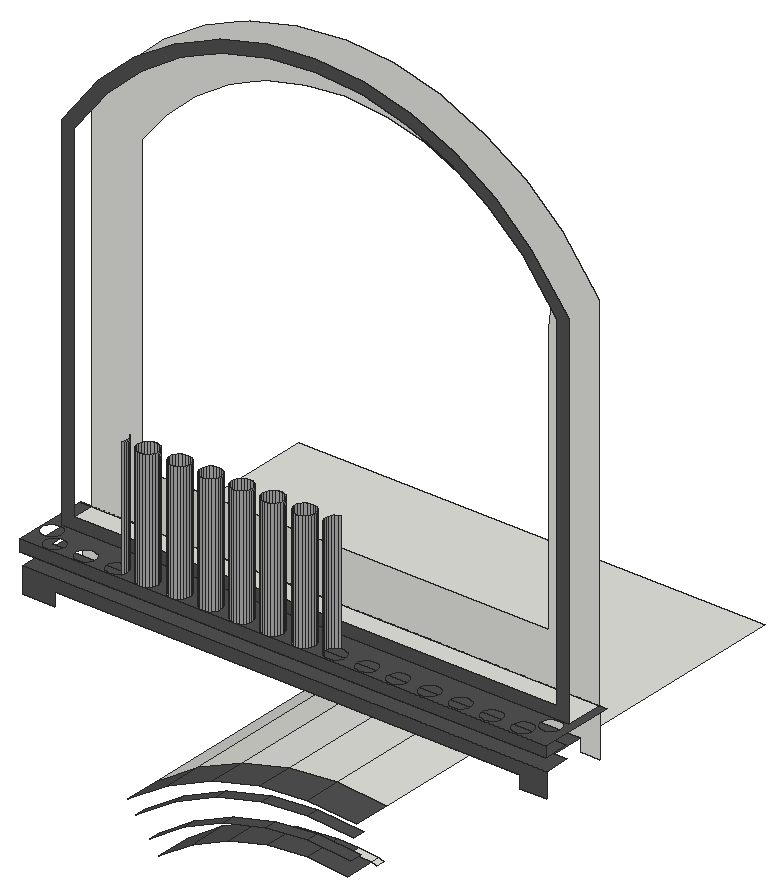
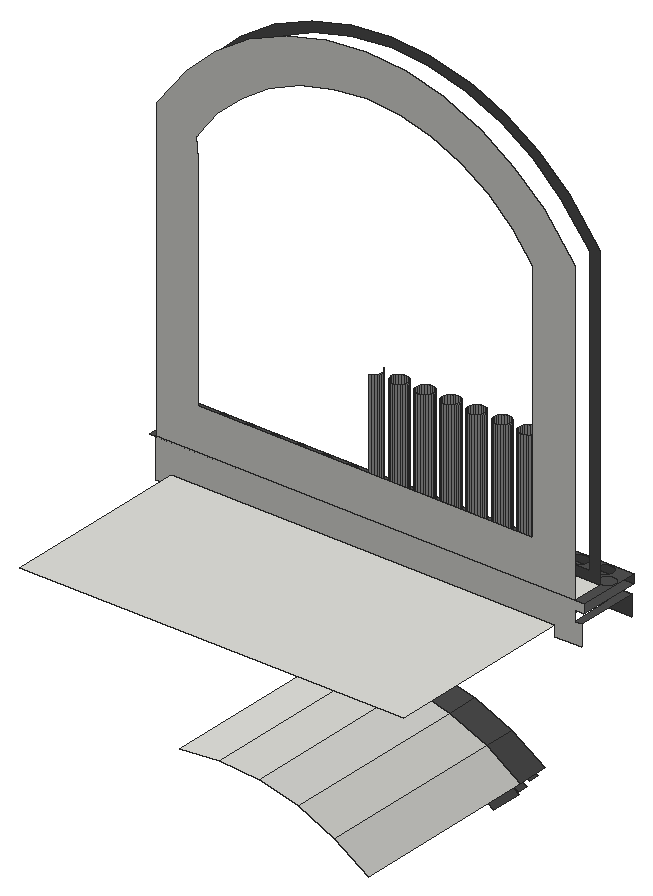
# SketchUp Ruby script. Lengths in inches.
U = 1.inch
M = Sketchup.active_model
def pt(a) = Geom::Point3d.new(a.map { |v| v * U })
def face(e, loops, mat)
  f = e.add_face(loops[0].map { |a| pt(a) })
  loops[1..].each { |l| e.add_face(l.map { |a| pt(a) }).erase! }
  f.material = f.back_material = mat if mat
  f
end
# faces: each face lists its corners as indices into pts; further lists are holes
def faces(e, pts, list, mat = nil) = list.each { |f| face(e, (f[0].is_a?(Array) ? f : [f]).map { |l| l.map { |i| pts[i] } }, mat) }
# xy, xz, yz: faces in a plane at the given z, y or x. An outline is a flat list of corners, or four numbers for a rectangle; further outlines are holes
def ring(l) = l.size == 4 ? [[l[0], l[1]], [l[2], l[1]], [l[2], l[3]], [l[0], l[3]]] : l.each_slice(2).to_a
def flat(e, list, mat, &to3) = list.each { |f| face(e, (f[0].is_a?(Array) ? f : [f]).map { |l| ring(l).map { |u, v| to3.(u, v) } }, mat) }
def xy(e, z, list, mat = nil) = flat(e, list, mat) { |x, y| [x, y, z] }
def xz(e, y, list, mat = nil) = flat(e, list, mat) { |x, z| [x, y, z] }
def yz(e, x, list, mat = nil) = flat(e, list, mat) { |y, z| [x, y, z] }
def lines(e, pts, list) = list.each { |a, b| e.add_line(pt(pts[a]), pt(pts[b])) }
# prism: a flat outline (further loops are holes) pulled along v
def prism(e, loops, v, mat = nil)
  f = face(e, loops, mat); d = Geom::Vector3d.new(v.map { |x| x * U })
  f.pushpull(f.normal.samedirection?(d) ? d.length : -d.length)
end
def box(e, o, s, mat = nil) = prism(e, [[o, [o[0] + s[0], o[1], o[2]], [o[0] + s[0], o[1] + s[1], o[2]], [o[0], o[1] + s[1], o[2]]]], [0, 0, s[2]], mat)
def at(x, y, z, deg = 0) = Geom::Transformation.translation(pt([x, y, z])) * Geom::Transformation.rotation(ORIGIN, Z_AXIS, deg.degrees)
def axes(o, x, y, z) = Geom::Transformation.new([*x, 0, *y, 0, *z, 0, *pt(o).to_a, 1])
def part(name) = M.definitions.add(name)
# library, detail: a bought-in or finely detailed component or shape, given as its bounding box
def library(name, o, s) = part(name).tap { |d| box(d.entities, o, s) }
def detail(e, o, s) = box(e.add_group.entities, o, s)
def put(e, d, t, mat = nil) = e.add_instance(d, t).tap { |i| i.material = mat if mat }
def group(e, t, mat = nil) = e.add_group.tap { |g| g.transformation = t; g.material = mat if mat }.entities
root = M.entities
M.materials.add("[0132_LightGray]").color = [169, 169, 169]
M.materials.add("[0135_DarkGray]").color = [81, 81, 81]
xy(root,487.28,[[247.74,49.6875,358.5,104.375]])
xy(root,487.28,[[247.74,31.6875,358.5,49.6875]],"[0135_DarkGray]")
xy(root,490.18,[[240.07,31.6875,364.76,31.6875,364.76,37.6875,242.14,37.6875,242.14,49.6875,240.07,49.6875]],"[0135_DarkGray]")
xy(root,493.07,[[239.45,31.6875,239.45,49.6875,242.14,49.6875,242.14,37.6875,364.64,37.6875,364.64,31.6875]],"[0135_DarkGray]")
xy(root,495.66,[[267.85,31.88,267.22,31.96,266.63,32.21,266.13,32.6,265.74,33.1,265.5,33.6875,265.41,34.32,265.5,34.95,265.74,35.54,266.13,36.04,266.63,36.43,267.22,36.67,267.85,36.76,268.48,36.67,269.07,36.43,269.58,36.04,269.96,35.54,270.21,34.95,270.29,34.32,270.21,33.6875,269.96,33.1,269.58,32.6,269.07,32.21,268.48,31.96],[275.29,31.88,274.66,31.96,274.07,32.21,273.57,32.6,273.18,33.1,272.93,33.6875,272.85,34.32,272.93,34.95,273.18,35.54,273.57,36.04,274.07,36.43,274.66,36.67,275.29,36.76,275.92,36.67,276.51,36.43,277.01,36.04,277.4,35.54,277.64,34.95,277.73,34.32,277.64,33.6875,277.4,33.1,277.01,32.6,276.51,32.21,275.92,31.96],[282.73,31.88,282.1,31.96,281.51,32.21,281,32.6,280.62,33.1,280.37,33.6875,280.29,34.32,280.37,34.95,280.62,35.54,281,36.04,281.51,36.43,282.1,36.67,282.73,36.76,283.36,36.67,283.95,36.43,284.45,36.04,284.84,35.54,285.08,34.95,285.16,34.32,285.08,33.6875,284.84,33.1,284.45,32.6,283.95,32.21,283.36,31.96],[290.16,31.88,289.53,31.96,288.95,32.21,288.44,32.6,288.05,33.1,287.81,33.6875,287.73,34.32,287.81,34.95,288.05,35.54,288.44,36.04,288.95,36.43,289.53,36.67,290.16,36.76,290.79,36.67,291.38,36.43,291.89,36.04,292.28,35.54,292.52,34.95,292.6,34.32,292.52,33.6875,292.28,33.1,291.89,32.6,291.38,32.21,290.79,31.96],[297.6,31.88,296.97,31.96,296.38,32.21,295.88,32.6,295.49,33.1,295.25,33.6875,295.16,34.32,295.25,34.95,295.49,35.54,295.88,36.04,296.38,36.43,296.97,36.67,297.6,36.76,298.23,36.67,298.82,36.43,299.33,36.04,299.71,35.54,299.96,34.95,300.04,34.32,299.96,33.6875,299.71,33.1,299.33,32.6,298.82,32.21,298.23,31.96],
  [305.04,31.88,304.41,31.96,303.82,32.21,303.32,32.6,302.93,33.1,302.68,33.6875,302.6,34.32,302.68,34.95,302.93,35.54,303.32,36.04,303.82,36.43,304.41,36.67,305.04,36.76,305.67,36.67,306.26,36.43,306.76,36.04,307.15,35.54,307.39,34.95,307.48,34.32,307.39,33.6875,307.15,33.1,306.76,32.6,306.26,32.21,305.67,31.96],[242.14,40.6875,362.82,49.6875]])
xy(root,495.66,[[[239.45,31.6875,364.64,31.6875,364.64,49.6875,362.82,49.6875,362.82,40.6875,242.14,40.6875,242.14,49.6875,239.45,49.6875],[245.54,31.88,244.91,31.96,244.32,32.21,243.82,32.6,243.43,33.1,243.18,33.6875,243.1,34.32,243.18,34.95,243.43,35.54,243.82,36.04,244.32,36.43,244.91,36.67,245.54,36.76,246.17,36.67,246.76,36.43,247.26,36.04,247.65,35.54,247.89,34.95,247.98,34.32,247.89,33.6875,247.65,33.1,247.26,32.6,246.76,32.21,246.17,31.96],[252.98,31.88,252.35,31.96,251.76,32.21,251.25,32.6,250.87,33.1,250.62,33.6875,250.54,34.32,250.62,34.95,250.87,35.54,251.25,36.04,251.76,36.43,252.35,36.67,252.98,36.76,253.61,36.67,254.2,36.43,254.7,36.04,255.09,35.54,255.33,34.95,255.41,34.32,255.33,33.6875,255.09,33.1,254.7,32.6,254.2,32.21,253.61,31.96],[260.41,31.88,259.78,31.96,259.2,32.21,258.69,32.6,258.3,33.1,258.06,33.6875,257.98,34.32,258.06,34.95,258.3,35.54,258.69,36.04,259.2,36.43,259.78,36.67,260.41,36.76,261.04,36.67,261.63,36.43,262.14,36.04,262.53,35.54,262.77,34.95,262.85,34.32,262.77,33.6875,262.53,33.1,262.14,32.6,261.63,32.21,261.04,31.96],[267.85,31.88,267.22,31.96,266.63,32.21,266.13,32.6,265.74,33.1,265.5,33.6875,265.41,34.32,265.5,34.95,265.74,35.54,266.13,36.04,266.63,36.43,267.22,36.67,267.85,36.76,268.48,36.67,269.07,36.43,269.58,36.04,269.96,35.54,270.21,34.95,270.29,34.32,270.21,33.6875,269.96,33.1,269.58,32.6,269.07,32.21,268.48,31.96],[275.29,31.88,274.66,31.96,274.07,32.21,273.57,32.6,273.18,33.1,272.93,33.6875,272.85,34.32,272.93,34.95,273.18,35.54,273.57,36.04,274.07,36.43,274.66,36.67,275.29,36.76,275.92,36.67,276.51,36.43,277.01,36.04,277.4,35.54,277.64,34.95,277.73,34.32,277.64,33.6875,277.4,33.1,277.01,32.6,276.51,32.21,275.92,31.96],[282.73,31.88,282.1,31.96,281.51,32.21,281,32.6,280.62,33.1,280.37,33.6875,280.29,34.32,280.37,34.95,280.62,35.54,281,36.04,281.51,36.43,282.1,36.67,282.73,36.76,283.36,36.67,283.95,36.43,284.45,36.04,284.84,35.54,285.08,34.95,285.16,34.32,285.08,33.6875,284.84,33.1,284.45,32.6,283.95,32.21,283.36,31.96],[290.16,31.88,289.53,31.96,288.95,32.21,288.44,32.6,288.05,33.1,287.81,33.6875,287.73,34.32,287.81,34.95,288.05,35.54,288.44,36.04,288.95,36.43,289.53,36.67,290.16,36.76,290.79,36.67,291.38,36.43,291.89,36.04,292.28,35.54,292.52,34.95,292.6,34.32,292.52,33.6875,292.28,33.1,291.89,32.6,291.38,32.21,290.79,31.96],[297.6,31.88,296.97,31.96,296.38,32.21,295.88,32.6,295.49,33.1,295.25,33.6875,295.16,34.32,295.25,34.95,295.49,35.54,295.88,36.04,296.38,36.43,296.97,36.67,297.6,36.76,298.23,36.67,298.82,36.43,299.33,36.04,299.71,35.54,299.96,34.95,300.04,34.32,299.96,33.6875,299.71,33.1,299.33,32.6,298.82,32.21,298.23,31.96],[305.04,31.88,304.41,31.96,303.82,32.21,303.32,32.6,302.93,33.1,302.68,33.6875,302.6,34.32,302.68,34.95,302.93,35.54,303.32,36.04,303.82,36.43,304.41,36.67,305.04,36.76,305.67,36.67,306.26,36.43,306.76,36.04,307.15,35.54,307.39,34.95,307.48,34.32,307.39,33.6875,307.15,33.1,306.76,32.6,306.26,32.21,305.67,31.96],[312.48,31.88,311.85,31.96,311.26,32.21,310.75,32.6,310.37,33.1,310.12,33.6875,310.04,34.32,310.12,34.95,310.37,35.54,310.75,36.04,311.26,36.43,311.85,36.67,312.48,36.76,313.11,36.67,313.7,36.43,314.2,36.04,314.59,35.54,314.83,34.95,314.91,34.32,314.83,33.6875,314.59,33.1,314.2,32.6,313.7,32.21,313.11,31.96],[319.91,31.88,319.28,31.96,318.7,32.21,318.19,32.6,317.8,33.1,317.56,33.6875,317.48,34.32,317.56,34.95,317.8,35.54,318.19,36.04,318.7,36.43,319.28,36.67,319.91,36.76,320.54,36.67,321.13,36.43,321.64,36.04,322.03,35.54,322.27,34.95,322.35,34.32,322.27,33.6875,322.03,33.1,321.64,32.6,321.13,32.21,320.54,31.96],[327.35,31.88,326.72,31.96,326.13,32.21,325.63,32.6,325.24,33.1,325,33.6875,324.91,34.32,325,34.95,325.24,35.54,325.63,36.04,326.13,36.43,326.72,36.67,327.35,36.76,327.98,36.67,328.57,36.43,329.08,36.04,329.46,35.54,329.71,34.95,329.79,34.32,329.71,33.6875,329.46,33.1,329.08,32.6,328.57,32.21,327.98,31.96],[334.79,31.88,334.16,31.96,333.57,32.21,333.07,32.6,332.68,33.1,332.43,33.6875,332.35,34.32,332.43,34.95,332.68,35.54,333.07,36.04,333.57,36.43,334.16,36.67,334.79,36.76,335.42,36.67,336.01,36.43,336.51,36.04,336.9,35.54,337.14,34.95,337.23,34.32,337.14,33.6875,336.9,33.1,336.51,32.6,336.01,32.21,335.42,31.96],[342.23,31.88,341.6,31.96,341.01,32.21,340.5,32.6,340.12,33.1,339.87,33.6875,339.79,34.32,339.87,34.95,340.12,35.54,340.5,36.04,341.01,36.43,341.6,36.67,342.23,36.76,342.86,36.67,343.45,36.43,343.95,36.04,344.34,35.54,344.58,34.95,344.66,34.32,344.58,33.6875,344.34,33.1,343.95,32.6,343.45,32.21,342.86,31.96],[349.66,31.88,349.03,31.96,348.45,32.21,347.94,32.6,347.55,33.1,347.31,33.6875,347.23,34.32,347.31,34.95,347.55,35.54,347.94,36.04,348.45,36.43,349.03,36.67,349.66,36.76,350.29,36.67,350.88,36.43,351.39,36.04,351.78,35.54,352.02,34.95,352.1,34.32,352.02,33.6875,351.78,33.1,351.39,32.6,350.88,32.21,350.29,31.96],[357.1,31.88,356.47,31.96,355.88,32.21,355.38,32.6,354.99,33.1,354.75,33.6875,354.66,34.32,354.75,34.95,354.99,35.54,355.38,36.04,355.88,36.43,356.47,36.67,357.1,36.76,357.73,36.67,358.32,36.43,358.83,36.04,359.21,35.54,359.46,34.95,359.54,34.32,359.46,33.6875,359.21,33.1,358.83,32.6,358.32,32.21,357.73,31.96],[360.59,35.72,359.96,35.81,359.37,36.05,358.86,36.4375,358.48,36.94,358.23,37.53,358.15,38.16,358.23,38.79,358.48,39.38,358.86,39.89,359.37,40.27,359.96,40.52,360.59,40.6,361.22,40.52,361.8,40.27,362.31,39.89,362.7,39.38,362.94,38.79,363.02,38.16,362.94,37.53,362.7,36.94,362.31,36.4375,361.8,36.05,361.22,35.81],[241.96,35.55,241.33,35.64,240.74,35.88,240.24,36.27,239.85,36.77,239.61,37.36,239.52,37.99,239.61,38.62,239.85,39.21,240.24,39.71,240.74,40.1,241.33,40.34,241.96,40.43,242.59,40.34,243.18,40.1,243.6875,39.71,244.07,39.21,244.32,38.62,244.4,37.99,244.32,37.36,244.07,36.77,243.6875,36.27,243.18,35.88,242.59,35.64]]],"[0135_DarkGray]")
xz(root,31.6875,[[240.07,484.28,247.74,484.28,247.74,487.28,358.5,487.28,358.5,484.28,364.76,484.28,364.76,490.18,240.07,490.18],[239.45,493.07,364.64,495.66]],"[0135_DarkGray]")
xz(root,40.6875,[[[242.14,495.66,362.82,495.66,362.82,582.07,353.9,593.68,345.43,601.54,335.77,607.9,328.81,610.98,325.2,612.57,314,615.43,302.48,616.39,290.96,615.43,279.76,612.57,276.15,610.98,269.18,607.9,259.53,601.54,251.0625,593.68,242.14,582.07],[244.93,498.46,244.93,581.12,253.14,591.78,261.26,599.34,270.53,605.4375,277.28,608.42,280.68,609.92,291.42,612.66,302.48,613.58,313.53,612.66,324.28,609.92,327.68,608.42,334.43,605.4375,343.69,599.34,351.82,591.78,360.02,581.12,360.02,498.46]]],"[0135_DarkGray]")
xz(root,49.6875,[[240.07,484.28,247.74,484.28,247.74,487.28,358.5,487.28,358.5,484.28,363.14,484.28,363.14,495.66,239.45,495.66,239.45,493.07,242.14,493.07,242.14,490.18,240.07,490.18],[[242.14,495.66,242.14,582.07,251.0625,593.68,259.53,601.54,269.18,607.9,276.15,610.98,279.76,612.57,290.96,615.43,302.48,616.39,314,615.43,325.2,612.57,328.81,610.98,335.77,607.9,345.43,601.54,353.9,593.68,362.82,582.07,362.82,495.66],[254.14,507.66,350.82,507.66,350.82,571.72,351.51,577.72,350.82,577.72,350.82,577.99,344.99,585.57,337.99,592.07,330.01,597.33,323.96,600,321.27,601.19,312,603.55,305.64,604.08,302.48,604.35,292.95,603.55,283.69,601.19,281,600,274.95,597.33,266.97,592.07,259.96,585.57,254.14,577.99]]])
p = [[265.28,49.6875,433.26],[273.26,49.6875,438.52],[273.26,40.6875,438.52],[265.28,40.6875,433.26],[271.56,43.6875,441.64],[263.08,43.6875,436.06],
  [263.08,40.6875,436.06],[271.56,40.6875,441.64],[282,49.6875,442.38],[282,40.6875,442.38],[259.88,43.6875,440.13],[269.08,43.6875,446.1875],
  [269.08,40.6875,446.1875],[259.88,40.6875,440.13],[280.84,43.6875,445.74],[280.84,40.6875,445.74],[291.27,49.6875,444.74],[291.27,40.6875,444.74],
  [267.5,49.6875,449.09],[257.84,49.6875,442.73],[257.84,40.6875,442.73],[267.5,40.6875,449.09],[257.84,104.375,442.73],[267.5,104.375,449.09],
  [310.32,49.6875,444.74],[311.64,49.6875,444.4],[311.64,47.6875,444.4],[310.32,47.6875,444.74],[300.79,49.6875,445.53],[300.79,40.6875,445.53],
  [305.64,49.6875,445.13],[305.64,47.6875,445.13],[310.32,40.6875,444.74],[290.68,43.6875,448.25],[290.68,40.6875,448.25],[279.15,43.6875,450.64],
  [279.15,40.6875,450.64],[300.79,43.6875,449.09],[300.79,40.6875,449.09],[310.91,43.6875,448.25],[310.91,40.6875,448.25],[278.07,49.6875,453.76],
  [278.07,40.6875,453.76],[278.07,104.375,453.76],[289.82,43.6875,453.36],[289.82,40.6875,453.36],[300.79,43.6875,454.27],[300.79,40.6875,454.27],
  [311.76,43.6875,453.36],[311.76,40.6875,453.36],[289.27,49.6875,456.61],[289.27,40.6875,456.61],[289.27,104.375,456.61],[300.79,49.6875,457.57],
  [300.79,40.6875,457.57],[312.3125,49.6875,456.61],[312.3125,40.6875,456.61],[300.79,104.375,457.57],[312.3125,104.375,456.61],[267.22,31.96,495.66],
  [267.85,31.88,495.66],[267.85,31.88,523.91],[267.22,31.96,523.91],[268.48,31.96,495.66],[268.48,31.96,523.91],[274.66,31.96,495.66],
  [275.29,31.88,495.66],[275.29,31.88,523.91],[274.66,31.96,523.91],[275.92,31.96,495.66],[275.92,31.96,523.91],[282.1,31.96,495.66],
  [282.73,31.88,495.66],[282.73,31.88,523.91],[282.1,31.96,523.91],[283.36,31.96,495.66],[283.36,31.96,523.91],[289.53,31.96,495.66],
  [290.16,31.88,495.66],[290.16,31.88,523.91],[289.53,31.96,523.91],[290.79,31.96,495.66],[290.79,31.96,523.91],[296.97,31.96,495.66],
  [297.6,31.88,495.66],[297.6,31.88,523.91],[296.97,31.96,523.91],[298.23,31.96,495.66],[298.23,31.96,523.91],[304.41,31.96,495.66],
  [305.04,31.88,495.66],[305.04,31.88,523.91],[304.41,31.96,523.91],[305.67,31.96,495.66],[305.67,31.96,523.91],[266.63,32.21,495.66],
  [266.63,32.21,523.91],[269.07,32.21,495.66],[269.07,32.21,523.91],[274.07,32.21,495.66],[274.07,32.21,523.91],[276.51,32.21,495.66],
  [276.51,32.21,523.91],[281.51,32.21,495.66],[281.51,32.21,523.91],[283.95,32.21,495.66],[283.95,32.21,523.91],[288.95,32.21,495.66],
  [288.95,32.21,523.91],[291.38,32.21,495.66],[291.38,32.21,523.91],[296.38,32.21,495.66],[296.38,32.21,523.91],[298.82,32.21,495.66],
  [298.82,32.21,523.91],[303.82,32.21,495.66],[303.82,32.21,523.91],[306.26,32.21,495.66],[306.26,32.21,523.91],[266.13,32.6,495.66],
  [266.13,32.6,523.91],[269.58,32.6,495.66],[269.58,32.6,523.91],[273.57,32.6,495.66],[273.57,32.6,523.91],[277.01,32.6,495.66],
  [277.01,32.6,523.91],[281,32.6,495.66],[281,32.6,523.91],[284.45,32.6,495.66],[284.45,32.6,523.91],[288.44,32.6,495.66],
  [288.44,32.6,523.91],[291.89,32.6,495.66],[291.89,32.6,523.91],[295.88,32.6,495.66],[295.88,32.6,523.91],[299.33,32.6,495.66],
  [299.33,32.6,523.91],[303.32,32.6,495.66],[303.32,32.6,523.91],[306.76,32.6,495.66],[306.76,32.6,523.91],[310.75,32.6,495.66],
  [311.26,32.21,495.66],[311.26,32.21,523.91],[310.75,32.6,523.91],[265.74,33.1,495.66],[265.74,33.1,523.91],[269.96,33.1,495.66],
  [269.96,33.1,523.91],[273.18,33.1,495.66],[273.18,33.1,523.91],[277.4,33.1,495.66],[277.4,33.1,523.91],[280.62,33.1,495.66],
  [280.62,33.1,523.91],[284.84,33.1,495.66],[284.84,33.1,523.91],[288.05,33.1,495.66],[288.05,33.1,523.91],[292.28,33.1,495.66],
  [292.28,33.1,523.91],[295.49,33.1,495.66],[295.49,33.1,523.91],[299.71,33.1,495.66],[299.71,33.1,523.91],[302.93,33.1,495.66],
  [302.93,33.1,523.91],[307.15,33.1,495.66],[307.15,33.1,523.91],[310.37,33.1,495.66],[310.37,33.1,523.91],[262.53,33.1,495.66],
  [262.77,33.6875,495.66],[262.77,33.6875,523.91],[262.53,33.1,523.91],[265.5,33.6875,495.66],[265.5,33.6875,523.91],[270.21,33.6875,495.66],
  [270.21,33.6875,523.91],[272.93,33.6875,495.66],[272.93,33.6875,523.91],[277.64,33.6875,495.66],[277.64,33.6875,523.91],[280.37,33.6875,495.66],
  [280.37,33.6875,523.91],[285.08,33.6875,495.66],[285.08,33.6875,523.91],[287.81,33.6875,495.66],[287.81,33.6875,523.91],[292.52,33.6875,495.66],
  [292.52,33.6875,523.91],[295.25,33.6875,495.66],[295.25,33.6875,523.91],[299.96,33.6875,495.66],[299.96,33.6875,523.91],[302.68,33.6875,495.66],
  [302.68,33.6875,523.91],[307.39,33.6875,495.66],[307.39,33.6875,523.91],[310.12,33.6875,495.66],[310.12,33.6875,523.91],[262.85,34.32,495.66],
  [262.85,34.32,523.91],[265.41,34.32,495.66],[265.41,34.32,523.91],[270.29,34.32,495.66],[270.29,34.32,523.91],[272.85,34.32,495.66],
  [272.85,34.32,523.91],[277.73,34.32,495.66],[277.73,34.32,523.91],[280.29,34.32,495.66],[280.29,34.32,523.91],[285.16,34.32,495.66],
  [285.16,34.32,523.91],[287.73,34.32,495.66],[287.73,34.32,523.91],[292.6,34.32,495.66],[292.6,34.32,523.91],[295.16,34.32,495.66],
  [295.16,34.32,523.91],[300.04,34.32,495.66],[300.04,34.32,523.91],[302.6,34.32,495.66],[302.6,34.32,523.91],[307.48,34.32,495.66],
  [307.48,34.32,523.91],[310.04,34.32,495.66],[310.04,34.32,523.91],[262.77,34.95,495.66],[262.77,34.95,523.91],[265.5,34.95,495.66],
  [265.5,34.95,523.91],[270.21,34.95,495.66],[270.21,34.95,523.91],[272.93,34.95,495.66],[272.93,34.95,523.91],[277.64,34.95,495.66],
  [277.64,34.95,523.91],[280.37,34.95,495.66],[280.37,34.95,523.91],[285.08,34.95,495.66],[285.08,34.95,523.91],[287.81,34.95,495.66],
  [287.81,34.95,523.91],[292.52,34.95,495.66],[292.52,34.95,523.91],[295.25,34.95,495.66],[295.25,34.95,523.91],[299.96,34.95,495.66],
  [299.96,34.95,523.91],[302.68,34.95,495.66],[302.68,34.95,523.91],[307.39,34.95,495.66],[307.39,34.95,523.91],[310.12,34.95,495.66],
  [310.12,34.95,523.91],[262.53,35.54,495.66],[262.53,35.54,523.91],[265.74,35.54,495.66],[265.74,35.54,523.91],[269.96,35.54,495.66],
  [269.96,35.54,523.91],[273.18,35.54,495.66],[273.18,35.54,523.91],[277.4,35.54,495.66],[277.4,35.54,523.91],[280.62,35.54,495.66],
  [280.62,35.54,523.91],[284.84,35.54,495.66],[284.84,35.54,523.91],[288.05,35.54,495.66],[288.05,35.54,523.91],[292.28,35.54,495.66],
  [292.28,35.54,523.91],[295.49,35.54,495.66],[295.49,35.54,523.91],[299.71,35.54,495.66],[299.71,35.54,523.91],[302.93,35.54,495.66],
  [302.93,35.54,523.91],[307.15,35.54,495.66],[307.15,35.54,523.91],[310.37,35.54,495.66],[310.37,35.54,523.91],[262.14,36.04,495.66],
  [262.14,36.04,523.91],[266.13,36.04,495.66],[266.13,36.04,523.91],[269.58,36.04,495.66],[269.58,36.04,523.91],[273.57,36.04,495.66],
  [273.57,36.04,523.91],[277.01,36.04,495.66],[277.01,36.04,523.91],[281,36.04,495.66],[281,36.04,523.91],[284.45,36.04,495.66],
  [284.45,36.04,523.91],[288.44,36.04,495.66],[288.44,36.04,523.91],[291.89,36.04,495.66],[291.89,36.04,523.91],[295.88,36.04,495.66],
  [295.88,36.04,523.91],[299.33,36.04,495.66],[299.33,36.04,523.91],[303.32,36.04,495.66],[303.32,36.04,523.91],[306.76,36.04,495.66],
  [306.76,36.04,523.91],[310.75,36.04,495.66],[310.75,36.04,523.91],[266.63,36.43,495.66],[266.63,36.43,523.91],[269.07,36.43,495.66],
  [269.07,36.43,523.91],[274.07,36.43,495.66],[274.07,36.43,523.91],[276.51,36.43,495.66],[276.51,36.43,523.91],[281.51,36.43,495.66],
  [281.51,36.43,523.91],[283.95,36.43,495.66],[283.95,36.43,523.91],[288.95,36.43,495.66],[288.95,36.43,523.91],[291.38,36.43,495.66],
  [291.38,36.43,523.91],[296.38,36.43,495.66],[296.38,36.43,523.91],[298.82,36.43,495.66],[298.82,36.43,523.91],[303.82,36.43,495.66],
  [303.82,36.43,523.91],[306.26,36.43,495.66],[306.26,36.43,523.91],[311.26,36.43,495.66],[311.26,36.43,523.91],[267.22,36.67,495.66],
  [267.22,36.67,523.91],[268.48,36.67,495.66],[268.48,36.67,523.91],[274.66,36.67,495.66],[274.66,36.67,523.91],[275.92,36.67,495.66],
  [275.92,36.67,523.91],[282.1,36.67,495.66],[282.1,36.67,523.91],[283.36,36.67,495.66],[283.36,36.67,523.91],[289.53,36.67,495.66],
  [289.53,36.67,523.91],[290.79,36.67,495.66],[290.79,36.67,523.91],[296.97,36.67,495.66],[296.97,36.67,523.91],[298.23,36.67,495.66],
  [298.23,36.67,523.91],[304.41,36.67,495.66],[304.41,36.67,523.91],[305.67,36.67,495.66],[305.67,36.67,523.91],[311.85,36.67,495.66],
  [311.85,36.67,523.91],[267.85,36.76,495.66],[267.85,36.76,523.91],[275.29,36.76,495.66],[275.29,36.76,523.91],[282.73,36.76,495.66],
  [282.73,36.76,523.91],[290.16,36.76,495.66],[290.16,36.76,523.91],[297.6,36.76,495.66],[297.6,36.76,523.91],[305.04,36.76,495.66],
  [305.04,36.76,523.91]]
faces(root,p,[[0,1,2,3],[4,5,6,7],[1,8,9,2],[10,11,12,13],[14,4,7,15],[8,16,17,9],[18,19,20,21],[16,28,29,17],
  [28,30,31,27,32,29],[33,14,15,34],[11,35,36,12],[37,33,34,38],[39,37,38,40],[41,18,21,42],[35,44,45,36],[44,46,47,45],
  [46,48,49,47],[50,41,42,51],[53,50,51,54],[55,53,54,56]],"[0135_DarkGray]")
faces(root,p,[[18,19,22,23],[24,25,26,27],[30,24,27,31],[41,18,23,43],[50,41,43,52],[53,50,52,57],[55,53,57,58]])
faces(root,p,[[59,60,61,62],[60,63,64,61],[65,66,67,68],[66,69,70,67],[71,72,73,74],[72,75,76,73],[77,78,79,80],[78,81,82,79],
  [83,84,85,86],[84,87,88,85],[89,90,91,92],[90,93,94,91],[95,59,62,96],[63,97,98,64],[99,65,68,100],[69,101,102,70],
  [103,71,74,104],[75,105,106,76],[107,77,80,108],[81,109,110,82],[111,83,86,112],[87,113,114,88],[115,89,92,116],[93,117,118,94],
  [119,95,96,120],[97,121,122,98],[123,99,100,124],[101,125,126,102],[127,103,104,128],[105,129,130,106],[131,107,108,132],[109,133,134,110],
  [135,111,112,136],[113,137,138,114],[139,115,116,140],[117,141,142,118],[143,144,145,146],[147,119,120,148],[121,149,150,122],[151,123,124,152],
  [125,153,154,126],[155,127,128,156],[129,157,158,130],[159,131,132,160],[133,161,162,134],[163,135,136,164],[137,165,166,138],[167,139,140,168],
  [141,169,170,142],[171,143,146,172],[173,174,175,176],[177,147,148,178],[149,179,180,150],[181,151,152,182],[153,183,184,154],[185,155,156,186],
  [157,187,188,158],[189,159,160,190],[161,191,192,162],[193,163,164,194],[165,195,196,166],[197,167,168,198],[169,199,200,170],[201,171,172,202],
  [174,203,204,175],[205,177,178,206],[179,207,208,180],[209,181,182,210],[183,211,212,184],[213,185,186,214],[187,215,216,188],[217,189,190,218],
  [191,219,220,192],[221,193,194,222],[195,223,224,196],[225,197,198,226],[199,227,228,200],[229,201,202,230],[203,231,232,204],[233,205,206,234],
  [207,235,236,208],[237,209,210,238],[211,239,240,212],[241,213,214,242],[215,243,244,216],[245,217,218,246],[219,247,248,220],[249,221,222,250],
  [223,251,252,224],[253,225,226,254],[227,255,256,228],[257,229,230,258],[231,259,260,232],[261,233,234,262],[235,263,264,236],[265,237,238,266],
  [239,267,268,240],[269,241,242,270],[243,271,272,244],[273,245,246,274],[247,275,276,248],[277,249,250,278],[251,279,280,252],[281,253,254,282],
  [255,283,284,256],[285,257,258,286],[259,287,288,260],[289,261,262,290],[263,291,292,264],[293,265,266,294],[267,295,296,268],[297,269,270,298],
  [271,299,300,272],[301,273,274,302],[275,303,304,276],[305,277,278,306],[279,307,308,280],[309,281,282,310],[283,311,312,284],[313,285,286,314],
  [315,289,290,316],[291,317,318,292],[319,293,294,320],[295,321,322,296],[323,297,298,324],[299,325,326,300],[327,301,302,328],[303,329,330,304],
  [331,305,306,332],[307,333,334,308],[335,309,310,336],[311,337,338,312],[339,313,314,340],[341,315,316,342],[317,343,344,318],[345,319,320,346],
  [321,347,348,322],[349,323,324,350],[325,351,352,326],[353,327,328,354],[329,355,356,330],[357,331,332,358],[333,359,360,334],[361,335,336,362],
  [337,363,364,338],[365,339,340,366],[367,341,342,368],[343,367,368,344],[369,345,346,370],[347,369,370,348],[371,349,350,372],[351,371,372,352],
  [373,353,354,374],[355,373,374,356],[375,357,358,376],[359,375,376,360],[377,361,362,378],[363,377,378,364]],"[0132_LightGray]")
